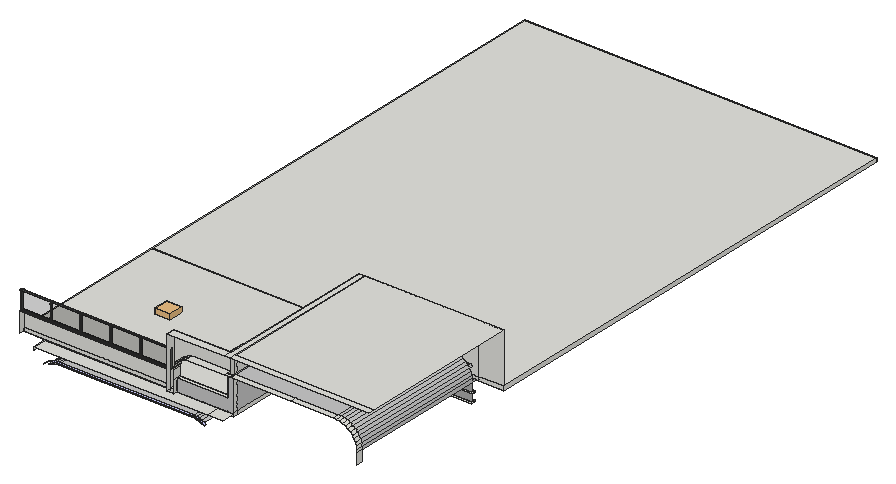
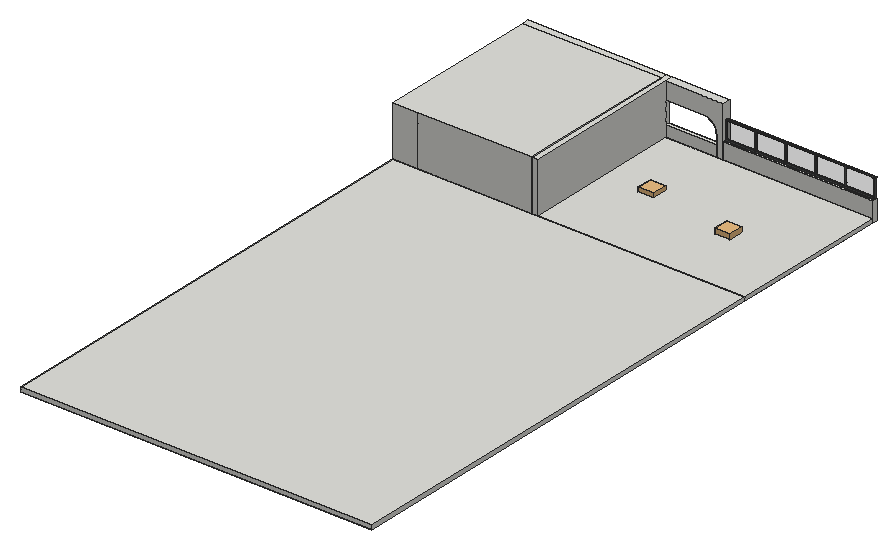
# SketchUp Ruby script. Lengths in inches.
U = 1.inch
M = Sketchup.active_model
def pt(a) = Geom::Point3d.new(a.map { |v| v * U })
def face(e, loops, mat)
  f = e.add_face(loops[0].map { |a| pt(a) })
  loops[1..].each { |l| e.add_face(l.map { |a| pt(a) }).erase! }
  f.material = f.back_material = mat if mat
  f
end
# faces: each face lists its corners as indices into pts; further lists are holes
def faces(e, pts, list, mat = nil) = list.each { |f| face(e, (f[0].is_a?(Array) ? f : [f]).map { |l| l.map { |i| pts[i] } }, mat) }
# xy, xz, yz: faces in a plane at the given z, y or x. An outline is a flat list of corners, or four numbers for a rectangle; further outlines are holes
def ring(l) = l.size == 4 ? [[l[0], l[1]], [l[2], l[1]], [l[2], l[3]], [l[0], l[3]]] : l.each_slice(2).to_a
def flat(e, list, mat, &to3) = list.each { |f| face(e, (f[0].is_a?(Array) ? f : [f]).map { |l| ring(l).map { |u, v| to3.(u, v) } }, mat) }
def xy(e, z, list, mat = nil) = flat(e, list, mat) { |x, y| [x, y, z] }
def xz(e, y, list, mat = nil) = flat(e, list, mat) { |x, z| [x, y, z] }
def yz(e, x, list, mat = nil) = flat(e, list, mat) { |y, z| [x, y, z] }
def lines(e, pts, list) = list.each { |a, b| e.add_line(pt(pts[a]), pt(pts[b])) }
# prism: a flat outline (further loops are holes) pulled along v
def prism(e, loops, v, mat = nil)
  f = face(e, loops, mat); d = Geom::Vector3d.new(v.map { |x| x * U })
  f.pushpull(f.normal.samedirection?(d) ? d.length : -d.length)
end
def box(e, o, s, mat = nil) = prism(e, [[o, [o[0] + s[0], o[1], o[2]], [o[0] + s[0], o[1] + s[1], o[2]], [o[0], o[1] + s[1], o[2]]]], [0, 0, s[2]], mat)
def at(x, y, z, deg = 0) = Geom::Transformation.translation(pt([x, y, z])) * Geom::Transformation.rotation(ORIGIN, Z_AXIS, deg.degrees)
def axes(o, x, y, z) = Geom::Transformation.new([*x, 0, *y, 0, *z, 0, *pt(o).to_a, 1])
def part(name) = M.definitions.add(name)
# library, detail: a bought-in or finely detailed component or shape, given as its bounding box
def library(name, o, s) = part(name).tap { |d| box(d.entities, o, s) }
def detail(e, o, s) = box(e.add_group.entities, o, s)
def put(e, d, t, mat = nil) = e.add_instance(d, t).tap { |i| i.material = mat if mat }
def group(e, t, mat = nil) = e.add_group.tap { |g| g.transformation = t; g.material = mat if mat }.entities
root = M.entities
M.materials.add("Aluminum_Polished").color = [83, 85, 85]
M.materials.add("Glass_Window_Neutral").color = [0, 0, 0]
M.materials["Glass_Window_Neutral"].alpha = 0.125
M.materials.add("[Color I01]").color = [204, 204, 255]
M.materials.add("[Color M02]").color = [198, 198, 198]
M.materials.add("[Color M03]").color = [170, 170, 170]
M.materials.add("[Color M06]").color = [86, 86, 86]
c1 = library("Omni Light\#2",[-12,-12,-12],[24,24,24])
c2 = library("Spot Light\#6",[-5.1,-5.1,-11.05],[10.2,10.2,11.05])
c3 = library("Omni Light\#1",[-12,-12,-12],[24,24,24])
c4 = library("Omni Light\#24",[-12,-12,-12],[24,24,24])
c5 = library("Spot Light\#10",[-5.1,-5.1,-11.05],[10.2,10.2,11.05])
c6 = part("Group\#54")
box(c6.entities,[0,0,0],[2,1,28])
c7 = part("Group\#56")
p = [[0.11,0.32,0.14],[0.11,0.69,0.14]]
lines(c7.entities,p,[[0,1]])
g1 = group(c7.entities,at(0.11,0,0))
prism(g1,[[[0,0.24,0],[0,0.32,0.14],[0,0.24,0.27],[0,0.08,0.27],[0,0,0.14],[0,0.08,0]]],[-0.11,0,0])
c8 = part("Ver Glass Railing")
g2 = group(c8.entities,at(0,0,0),"Aluminum_Polished")
box(g2,[0,0,0],[2,185,2])
g3 = group(c8.entities,at(0,0,2),"Aluminum_Polished")
p = [[1.41,1,0],[1.41,36.8,0],[1.41,184,0],[1.29,184,0],[1.29,1,0],[1.29,36.8,0],
  [1.41,184,28],[1.29,184,28],[1.41,148.2,28],[1.29,148.2,28],[1.41,1,28],[1.29,1,28],
  [1.29,111.4,28],[1.29,111.4,0],[1.41,111.4,0],[1.41,111.4,28],[1.29,110.4,0],[1.29,110.4,28],
  [1.41,110.4,28],[1.41,110.4,0],[1.29,74.6,28],[1.29,74.6,0],[1.41,74.6,0],[1.41,74.6,28],
  [1.29,73.6,0],[1.29,73.6,28],[1.41,73.6,28],[1.41,73.6,0],[1.29,148.2,0],[1.41,148.2,0],
  [1.29,147.2,0],[1.29,147.2,28],[1.41,147.2,28],[1.41,147.2,0],[1.29,37.8,28],[1.29,37.8,0],
  [1.41,37.8,0],[1.41,37.8,28],[1.29,36.8,28],[1.41,36.8,28]]
lines(g3,p,[[0,1],[2,3],[4,5],[6,7],[6,8],[7,9],[10,11],[2,6],[3,7],[0,4],[11,4],[10,0],
  [12,13],[14,15],[16,17],[18,19],[20,21],[22,23],[24,25],[26,27],[27,22],[24,21],[23,26],[20,25],
  [9,28],[29,8],[30,31],[32,33],[33,29],[30,28],[8,32],[9,31],[34,35],[36,37],[5,38],[39,1],
  [1,36],[5,35],[37,39],[14,33],[19,14],[22,19],[36,27],[13,30],[16,13],[21,16],[35,24],[15,18],
  [12,17],[29,2],[28,3],[18,23],[32,15],[17,20],[31,12],[26,37],[25,34],[34,38],[39,10],[38,11]])
g4 = group(g3,at(1.79,1,0))
box(g4,[-0.5,0,0],[0.125,183,28],"Glass_Window_Neutral")
g5 = group(g3,at(0,184,28))
box(g5,[0,-184,0],[2.5,185,1])
put(g3,c6,axes([2,185,28],[-1,0,0],[0,-1,0],[0,0,-1]))
put(g3,c6,axes([2,1,28],[-1,0,0],[0,-1,0],[0,0,-1]))
put(g3,c6,axes([2,111.4,28],[-1,0,0],[0,-1,0],[0,0,-1]))
put(g3,c6,axes([2,74.6,28],[-1,0,0],[0,-1,0],[0,0,-1]))
g6 = group(g3,at(2,148.2,28))
box(g6,[-2,-1,-28],[2,1,28])
put(g3,c6,axes([2,37.8,28],[-1,0,0],[0,-1,0],[0,0,-1]))
put(g3,c7,at(1.17,146.31,24.26))
put(g3,c7,axes([1.17,148.89,24.54],[1,0,0],[0,-1,0],[0,0,-1]))
put(g3,c7,axes([1.17,148.89,4.79],[1,0,0],[0,-1,0],[0,0,-1]))
put(g3,c7,at(1.17,146.31,4.51))
put(g3,c7,at(1.17,109.51,4.51))
put(g3,c7,axes([1.17,112.09,4.79],[1,0,0],[0,-1,0],[0,0,-1]))
put(g3,c7,axes([1.17,112.09,24.54],[1,0,0],[0,-1,0],[0,0,-1]))
put(g3,c7,at(1.17,109.51,24.26))
put(g3,c7,axes([1.17,75.29,24.54],[1,0,0],[0,-1,0],[0,0,-1]))
put(g3,c7,at(1.17,72.71,4.51))
put(g3,c7,axes([1.17,75.29,4.79],[1,0,0],[0,-1,0],[0,0,-1]))
put(g3,c7,at(1.17,72.71,24.26))
put(g3,c7,axes([1.17,38.49,24.54],[1,0,0],[0,-1,0],[0,0,-1]))
put(g3,c7,at(1.17,35.91,4.51))
put(g3,c7,axes([1.17,38.49,4.79],[1,0,0],[0,-1,0],[0,0,-1]))
put(g3,c7,at(1.17,35.91,24.26))
c9 = library("Omni Light\#10",[-12,-12,-12],[24,24,24])
xy(root,236.41,[[128.55,200.3125,339.27,237.125]],"[Color M02]")
xy(root,237.98,[[390.47,440.75,591.56,446.25]])
xy(root,240.67,[[390.47,440.75,591.56,446.25]])
xy(root,246,[[91.81,197.75,91.94,219.25],[91.81,219.25,91.94,225.88],[91.94,219.25,366.43,225.88],[366.43,219.25,390.47,225.88],[52.9375,225.88,91.81,440.75],
  [91.81,225.88,91.94,237.125],[91.94,225.88,390.47,237.125],[91.81,237.125,91.94,440.75],[52.9375,440.75,91.94,479.76],[91.94,440.75,390.47,479.76],
  [52.9375,479.76,91.94,479.76,91.94,1178.18,571.24,1178.18,571.24,479.76,610.25,479.76,610.25,1217.1875,52.9375,1217.1875],[91.94,479.76,571.24,1178.18]])
xy(root,246,[[[91.94,237.125,390.47,440.75],[173.35,341.64,176.46,342.05,179.35,343.24,181.83,345.15,183.74,347.64,184.94,350.53,185.35,353.64,184.94,356.74,183.74,359.64,181.83,362.12,179.35,364.03,176.46,365.23,173.35,365.64,170.24,365.23,167.35,364.03,164.86,362.12,162.96,359.64,161.76,356.74,161.35,353.64,161.76,350.53,162.96,347.64,164.86,345.15,167.35,343.24,170.24,342.05],[310.54,341.64,313.65,342.05,316.54,343.24,319.02,345.15,320.93,347.64,322.13,350.53,322.54,353.64,322.13,356.74,320.93,359.64,319.02,362.12,316.54,364.03,313.65,365.23,310.54,365.64,307.43,365.23,304.54,364.03,302.05,362.12,300.15,359.64,298.95,356.74,298.54,353.64,298.95,350.53,300.15,347.64,302.05,345.15,304.54,343.24,307.43,342.05]]],"[Color M02]")
xy(root,247.5625,[[173.35,341.64,170.24,342.05,167.35,343.24,164.86,345.15,162.96,347.64,161.76,350.53,161.35,353.64,161.76,356.74,162.96,359.64,164.86,362.12,167.35,364.03,170.24,365.23,173.35,365.64,176.46,365.23,179.35,364.03,181.83,362.12,183.74,359.64,184.94,356.74,185.35,353.64,184.94,350.53,183.74,347.64,181.83,345.15,179.35,343.24,176.46,342.05],[310.54,341.64,307.43,342.05,304.54,343.24,302.05,345.15,300.15,347.64,298.95,350.53,298.54,353.64,298.95,356.74,300.15,359.64,302.05,362.12,304.54,364.03,307.43,365.23,310.54,365.64,313.65,365.23,316.54,364.03,319.02,362.12,320.93,359.64,322.13,356.74,322.54,353.64,322.13,350.53,320.93,347.64,319.02,345.15,316.54,343.24,313.65,342.05]])
xy(root,249.875,[[91.94,197.75,366.43,197.75,366.43,219.25,300.96,219.25,300.96,213,290.41,213,290.41,219.25,91.94,219.25],[366.43,197.75,390.47,219.25]])
xy(root,252,[[290.41,219.25,300.96,225.88],[52.9375,225.88,381.14,479.76],[381.14,225.88,390.47,479.76],[52.9375,479.76,610.25,1217.1875]])
xy(root,267.76,[[390.47,440.75,591.56,446.25]])
xy(root,269.5,[[300.96,219.25,381.14,225.88]])
xy(root,270.45,[[390.47,440.75,591.38,446.25]])
xy(root,277.0625,[[52.9375,219.25,290.41,225.88]])
xy(root,286.19,[[390.47,440.75,586.62,446.25]])
xy(root,288.88,[[390.47,440.75,584.82,446.25]])
xy(root,304.625,[[320.39,213,381.14,225.88],[381.14,213,390.47,219.25],[390.47,213,486.31,222.9375],[486.31,213,554.68,222.9375]])
xy(root,304.625,[[390.47,222.9375,554.68,440.75]],"[Color M02]")
xy(root,331.6875,[[290.41,213,381.14,225.88],[381.14,213,390.47,479.76],[390.47,213,610.25,222.9375],[390.47,222.9375,610.25,479.76]])
xz(root,219.25,[[91.94,246,290.41,249.875],[290.41,246,300.96,252],[300.96,246,366.43,249.875],[366.43,246,390.47,249.875]])
xz(root,219.25,[[300.96,249.875,390.47,249.875,390.47,304.625,381.14,304.625,381.14,269.5,300.96,269.5]],"[Color M02]")
xz(root,225.88,[[52.9375,246,390.47,252],[52.9375,252,290.41,277.0625],[290.41,252,290.41,331.6875,381.14,331.6875,381.14,304.625,320.39,304.625,317.79,304.26,315.27,303.58,312.84,302.58,310.5625,301.3,308.46,299.74,306.5625,297.93,304.91,295.9,303.52,293.68,302.41,291.31,301.61,288.8125,301.125,286.24,300.96,283.625,300.96,252],[300.96,252,381.14,269.5]])
xz(root,440.75,[[390.47,240.67,591.56,240.67,591.56,251.38,390.47,252],[591.56,254.07,591.56,267.76,390.47,267.76,390.47,254.6875],[390.47,270.45,591.38,270.45,591.24,272.57,590.3,277.3,588.75,281.87,586.62,286.19,390.47,286.19],[390.47,288.88,584.82,288.88,583.9375,290.2,580.76,293.83,577.13,297.01,573.12,299.6875,568.79,301.82,564.23,303.37,559.5,304.31,554.68,304.625,390.47,304.625]],"[Color M03]")
xz(root,446.25,[[390.47,237.98,591.56,240.67],[591.56,251.38,591.56,254.07,390.47,254.6875,390.47,252],[390.47,267.76,591.56,267.76,591.38,270.45,390.47,270.45],[390.47,286.19,586.62,286.19,584.82,288.88,390.47,288.88]],"[Color M06]")
xz(root,479.76,[[52.9375,246,381.14,252],[381.14,246,390.47,252],[390.47,246,571.24,252],[571.24,246,610.25,252],[381.14,252,390.47,331.6875],
  [390.47,252,571.24,331.6875],[571.24,252,610.25,331.6875]])
xz(root,1217.1875,[[52.9375,246,610.25,252]])
yz(root,52.9375,[[219.25,246,225.88,277.0625],[225.88,246,479.76,252],[479.76,246,1217.1875,252]])
yz(root,91.94,[[197.75,246,219.25,249.875]])
yz(root,290.41,[[213,249.875,213,331.6875,225.88,331.6875,225.88,277.0625,219.25,277.0625,219.25,249.875],[219.25,252,225.88,277.0625]])
yz(root,300.96,[[213,249.875,219.25,269.5],[219.25,252,225.88,269.5],[213,269.5,225.88,283.625]])
yz(root,381.14,[[225.88,252,479.76,331.6875],[219.25,269.5,225.88,304.625]])
yz(root,390.47,[[440.75,237.98,446.25,240.67],[219.25,246,225.88,252],[225.88,246,440.75,252],[440.75,246,479.76,252],[219.25,252,225.88,304.625],
  [446.25,252,479.76,252,479.76,304.625,440.75,304.625,440.75,288.88,446.25,288.88,446.25,286.19,440.75,286.19,440.75,270.45,446.25,270.45,446.25,267.76,440.75,267.76,440.75,254.6875,446.25,254.6875],[222.9375,304.625,225.88,331.6875],[225.88,304.625,440.75,331.6875],[440.75,304.625,479.76,331.6875]])
yz(root,390.47,[[225.88,252,446.25,252,446.25,254.6875,440.75,254.6875,440.75,267.76,446.25,267.76,446.25,270.45,440.75,270.45,440.75,286.19,446.25,286.19,446.25,288.88,440.75,288.88,440.75,304.625,225.88,304.625]],"[Color M02]")
yz(root,591.56,[[213,251.38,222.9375,267.76]])
yz(root,610.25,[[479.76,246,1217.1875,252]])
p = [[115.63,237.125,232.95],[115.63,200.3125,232.95],[112.82,200.3125,231.07],[112.82,237.125,231.07],[110.49,197.75,234.11],[107.57,197.75,231.55],
  [107.57,200.3125,231.55],[110.49,200.3125,234.11],[356.11,237.125,231.9],[356.11,200.3125,231.9],[352.16,200.3125,233.85],[352.16,237.125,233.85],
  [362.11,197.75,232.49],[358.03,197.75,235.21],[358.03,200.3125,235.21],[362.11,200.3125,232.49],[118.66,237.125,234.44],[118.66,200.3125,234.44],
  [347.99,200.3125,235.26],[347.99,237.125,235.26],[113.71,197.75,236.26],[113.71,200.3125,236.26],[121.86,237.125,235.53],[121.86,200.3125,235.53],
  [353.625,197.75,237.38],[353.625,200.3125,237.38],[343.66,200.3125,236.12],[343.66,237.125,236.12],[125.18,237.125,236.19],[125.18,200.3125,236.19],
  [339.27,200.3125,236.41],[339.27,237.125,236.41],[128.55,237.125,236.41],[128.55,200.3125,236.41],[117.19,197.75,237.98],[117.19,200.3125,237.98],
  [348.98,197.75,238.96],[348.98,200.3125,238.96],[120.87,197.75,239.23],[120.87,200.3125,239.23],[344.16,197.75,239.92],[344.16,200.3125,239.92],
  [124.68,197.75,239.99],[124.68,200.3125,239.99],[339.27,197.75,240.24],[339.27,200.3125,240.24],[173.35,341.64,246],[170.24,342.05,246],
  [170.24,342.05,247.5625],[173.35,341.64,247.5625],[176.46,342.05,246],[176.46,342.05,247.5625],[310.54,341.64,246],[307.43,342.05,246],
  [307.43,342.05,247.5625],[310.54,341.64,247.5625],[313.65,342.05,246],[313.65,342.05,247.5625],[167.35,343.24,246],[167.35,343.24,247.5625],
  [179.35,343.24,246],[179.35,343.24,247.5625],[304.54,343.24,246],[304.54,343.24,247.5625],[316.54,343.24,246],[316.54,343.24,247.5625],
  [164.86,345.15,246],[164.86,345.15,247.5625],[181.83,345.15,246],[181.83,345.15,247.5625],[302.05,345.15,246],[302.05,345.15,247.5625],
  [319.02,345.15,246],[319.02,345.15,247.5625],[162.96,347.64,246],[162.96,347.64,247.5625],[183.74,347.64,246],[183.74,347.64,247.5625],
  [300.15,347.64,246],[300.15,347.64,247.5625],[320.93,347.64,246],[320.93,347.64,247.5625],[161.76,350.53,246],[161.76,350.53,247.5625],
  [184.94,350.53,246],[184.94,350.53,247.5625],[298.95,350.53,246],[298.95,350.53,247.5625],[322.13,350.53,246],[322.13,350.53,247.5625],
  [161.35,353.64,246],[161.35,353.64,247.5625],[185.35,353.64,246],[185.35,353.64,247.5625],[298.54,353.64,246],[298.54,353.64,247.5625],
  [322.54,353.64,246],[322.54,353.64,247.5625],[161.76,356.74,246],[161.76,356.74,247.5625],[184.94,356.74,246],[184.94,356.74,247.5625],
  [298.95,356.74,246],[298.95,356.74,247.5625],[322.13,356.74,246],[322.13,356.74,247.5625],[162.96,359.64,246],[162.96,359.64,247.5625],
  [183.74,359.64,246],[183.74,359.64,247.5625],[300.15,359.64,246],[300.15,359.64,247.5625],[320.93,359.64,246],[320.93,359.64,247.5625],
  [164.86,362.12,246],[164.86,362.12,247.5625],[181.83,362.12,246],[181.83,362.12,247.5625],[302.05,362.12,246],[302.05,362.12,247.5625],
  [319.02,362.12,246],[319.02,362.12,247.5625],[167.35,364.03,246],[167.35,364.03,247.5625],[179.35,364.03,246],[179.35,364.03,247.5625],
  [304.54,364.03,246],[304.54,364.03,247.5625],[316.54,364.03,246],[316.54,364.03,247.5625],[170.24,365.23,246],[170.24,365.23,247.5625],
  [176.46,365.23,246],[176.46,365.23,247.5625],[307.43,365.23,246],[307.43,365.23,247.5625],[313.65,365.23,246],[313.65,365.23,247.5625],
  [173.35,365.64,246],[173.35,365.64,247.5625],[310.54,365.64,246],[310.54,365.64,247.5625],[390.47,440.75,252],[591.56,440.75,251.38],
  [591.56,446.25,251.38],[390.47,446.25,252],[591.56,440.75,254.07],[390.47,440.75,254.6875],[390.47,446.25,254.6875],[591.56,446.25,254.07],
  [591.56,222.9375,267.76],[591.56,213,267.76],[591.24,213,272.57],[591.24,222.9375,272.57],[591.24,440.75,272.57],[591.38,440.75,270.45],
  [591.38,446.25,270.45],[591.56,446.25,267.76],[591.56,440.75,267.76],[590.3,213,277.3],[590.3,222.9375,277.3],[590.3,440.75,277.3],
  [588.75,213,281.87],[588.75,222.9375,281.87],[588.75,440.75,281.87],[586.62,213,286.19],[586.62,222.9375,286.19],[586.62,440.75,286.19],
  [301.125,225.88,286.24],[301.125,213,286.24],[300.96,213,283.625],[300.96,225.88,283.625],[301.61,225.88,288.8125],[301.61,213,288.8125],
  [583.9375,213,290.2],[583.9375,222.9375,290.2],[583.9375,440.75,290.2],[584.82,440.75,288.88],[584.82,446.25,288.88],[586.62,446.25,286.19],
  [302.41,225.88,291.31],[302.41,213,291.31],[580.76,213,293.83],[580.76,222.9375,293.83],[580.76,440.75,293.83],[303.52,225.88,293.68],
  [303.52,213,293.68],[304.91,225.88,295.9],[304.91,213,295.9],[577.13,213,297.01],[577.13,222.9375,297.01],[577.13,440.75,297.01],
  [306.5625,225.88,297.93],[306.5625,213,297.93],[573.12,213,299.6875],[573.12,222.9375,299.6875],[573.12,440.75,299.6875],[308.46,225.88,299.74],
  [308.46,213,299.74],[310.5625,225.88,301.3],[310.5625,213,301.3],[568.79,213,301.82],[568.79,222.9375,301.82],[568.79,440.75,301.82],
  [312.84,225.88,302.58],[312.84,213,302.58],[564.23,213,303.37],[564.23,222.9375,303.37],[564.23,440.75,303.37],[315.27,225.88,303.58],
  [315.27,213,303.58],[559.5,213,304.31],[559.5,222.9375,304.31],[559.5,440.75,304.31],[317.79,225.88,304.26],[317.79,213,304.26],
  [320.39,225.88,304.625],[320.39,213,304.625],[554.68,213,304.625],[554.68,222.9375,304.625],[554.68,440.75,304.625],[381.14,219.25,252],
  [381.14,225.88,252],[591.56,440.75,270.45],[586.62,440.75,288.88],[128.55,197.75,240.24]]
faces(root,p,[[0,1,2,3],[8,9,10,11],[16,17,1,0],[11,10,18,19],[22,23,17,16],[19,18,26,27],[28,29,23,22],[27,26,30,31],
  [32,33,29,28],[154,155,156,157,158,150,153],[161,154,153,160],[164,161,160,163],[167,164,163,166],[176,177,178,179,167,166,175],[184,176,175,183],[191,184,183,190],
  [196,191,190,195],[203,196,195,202],[208,203,202,207],[213,208,207,212],[220,213,212,219]],"[Color M02]")
faces(root,p,[[4,5,6,7],[12,13,14,15],[20,4,7,21],[13,24,25,14],[34,20,21,35],[24,36,37,25],[38,34,35,39],[36,40,41,37],
  [42,38,39,43],[40,44,45,41],[44,42,43,45]],"[Color I01]")
faces(root,p,[[46,47,48,49],[50,46,49,51],[52,53,54,55],[56,52,55,57],[47,58,59,48],[60,50,51,61],[53,62,63,54],[64,56,57,65],
  [58,66,67,59],[68,60,61,69],[62,70,71,63],[72,64,65,73],[66,74,75,67],[76,68,69,77],[70,78,79,71],[80,72,73,81],
  [74,82,83,75],[84,76,77,85],[78,86,87,79],[88,80,81,89],[82,90,91,83],[92,84,85,93],[86,94,95,87],[96,88,89,97],
  [90,98,99,91],[100,92,93,101],[94,102,103,95],[104,96,97,105],[98,106,107,99],[108,100,101,109],[102,110,111,103],[112,104,105,113],
  [106,114,115,107],[116,108,109,117],[110,118,119,111],[120,112,113,121],[114,122,123,115],[124,116,117,125],[118,126,127,119],[128,120,121,129],
  [122,130,131,123],[132,124,125,133],[126,134,135,127],[136,128,129,137],[130,138,139,131],[138,132,133,139],[134,140,141,135],[140,136,137,141],
  [142,143,144,145],[146,147,148,149],[150,151,152,153],[153,152,159,160],[160,159,162,163],[163,162,165,166],[168,169,170,171],[172,173,169,168],
  [166,165,174,175],[180,181,173,172],[175,174,182,183],[185,186,181,180],[187,188,186,185],[183,182,189,190],[192,193,188,187],[190,189,194,195],
  [197,198,193,192],[199,200,198,197],[195,194,201,202],[204,205,200,199],[202,201,206,207],[209,210,205,204],[207,206,211,212],[214,215,210,209],
  [216,217,215,214],[212,211,218,219]])
lines(root,p,[[221,222],[223,155],[224,177],[225,42]])
put(root,c1,at(310.54,341.64,246))
put(root,c2,at(307.43,342.05,246))
put(root,c3,at(170.24,365.23,247.5625))
put(root,c4,at(495.75,327.98,275.7))
put(root,c5,axes([486.26,328.98,293.5625],[1.87,0,0],[0,1.87,0],[0,0,1.87]))
put(root,c8,axes([52.9375,221.75,277.0625],[0,-1,0],[1.28364,0,0],[0,0,1]))
put(root,c9,at(482.89,334.38,293.57))
